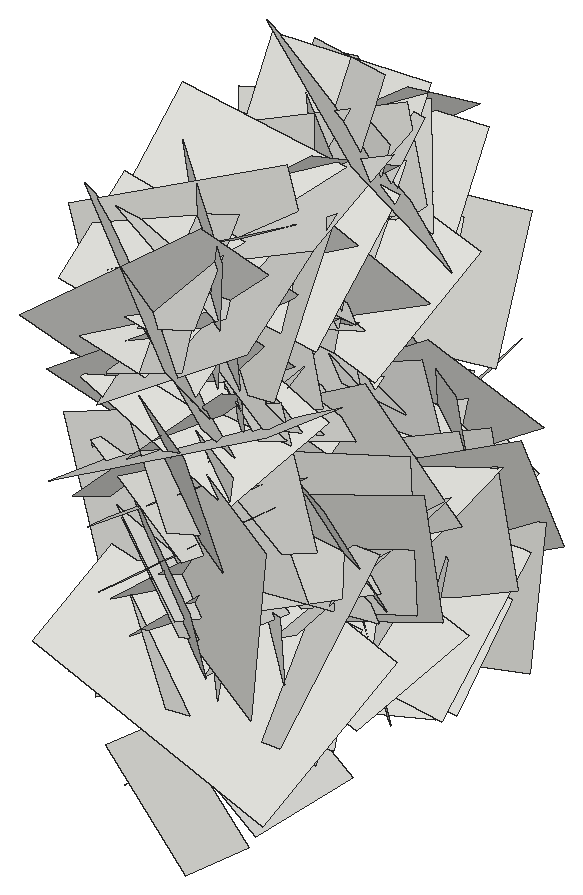
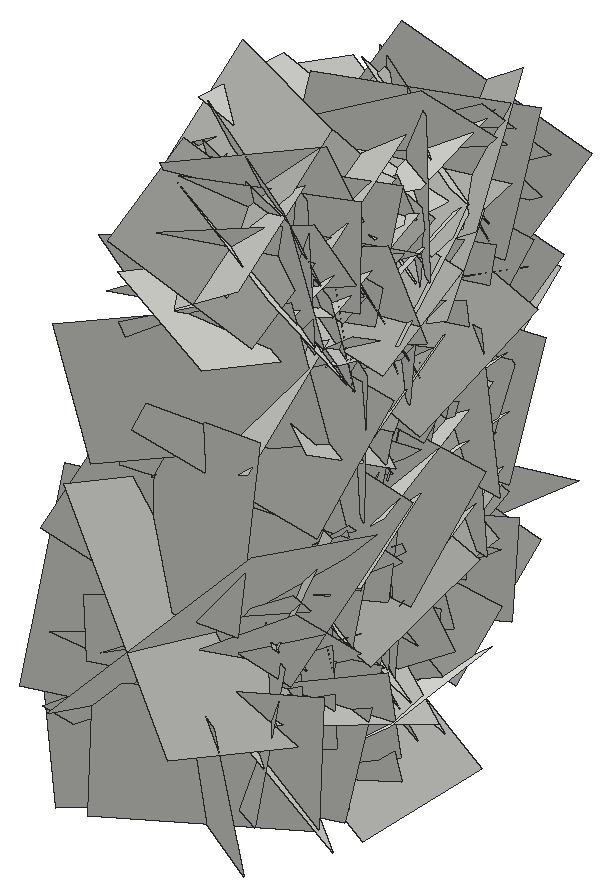
# SketchUp Ruby script. Lengths in inches.
U = 1.inch
M = Sketchup.active_model
def pt(a) = Geom::Point3d.new(a.map { |v| v * U })
def face(e, loops, mat)
  f = e.add_face(loops[0].map { |a| pt(a) })
  loops[1..].each { |l| e.add_face(l.map { |a| pt(a) }).erase! }
  f.material = f.back_material = mat if mat
  f
end
# faces: each face lists its corners as indices into pts; further lists are holes
def faces(e, pts, list, mat = nil) = list.each { |f| face(e, (f[0].is_a?(Array) ? f : [f]).map { |l| l.map { |i| pts[i] } }, mat) }
# xy, xz, yz: faces in a plane at the given z, y or x. An outline is a flat list of corners, or four numbers for a rectangle; further outlines are holes
def ring(l) = l.size == 4 ? [[l[0], l[1]], [l[2], l[1]], [l[2], l[3]], [l[0], l[3]]] : l.each_slice(2).to_a
def flat(e, list, mat, &to3) = list.each { |f| face(e, (f[0].is_a?(Array) ? f : [f]).map { |l| ring(l).map { |u, v| to3.(u, v) } }, mat) }
def xy(e, z, list, mat = nil) = flat(e, list, mat) { |x, y| [x, y, z] }
def xz(e, y, list, mat = nil) = flat(e, list, mat) { |x, z| [x, y, z] }
def yz(e, x, list, mat = nil) = flat(e, list, mat) { |y, z| [x, y, z] }
def lines(e, pts, list) = list.each { |a, b| e.add_line(pt(pts[a]), pt(pts[b])) }
# prism: a flat outline (further loops are holes) pulled along v
def prism(e, loops, v, mat = nil)
  f = face(e, loops, mat); d = Geom::Vector3d.new(v.map { |x| x * U })
  f.pushpull(f.normal.samedirection?(d) ? d.length : -d.length)
end
def box(e, o, s, mat = nil) = prism(e, [[o, [o[0] + s[0], o[1], o[2]], [o[0] + s[0], o[1] + s[1], o[2]], [o[0], o[1] + s[1], o[2]]]], [0, 0, s[2]], mat)
def at(x, y, z, deg = 0) = Geom::Transformation.translation(pt([x, y, z])) * Geom::Transformation.rotation(ORIGIN, Z_AXIS, deg.degrees)
def axes(o, x, y, z) = Geom::Transformation.new([*x, 0, *y, 0, *z, 0, *pt(o).to_a, 1])
def part(name) = M.definitions.add(name)
# library, detail: a bought-in or finely detailed component or shape, given as its bounding box
def library(name, o, s) = part(name).tap { |d| box(d.entities, o, s) }
def detail(e, o, s) = box(e.add_group.entities, o, s)
def put(e, d, t, mat = nil) = e.add_instance(d, t).tap { |i| i.material = mat if mat }
def group(e, t, mat = nil) = e.add_group.tap { |g| g.transformation = t; g.material = mat if mat }.entities
root = M.entities
c1 = part("Component\#6")
p = [[0.01,0,0],[0,3.24,4.54],[4.32,3.24,4.54],[4.33,0,0]]
faces(c1.entities,p,[[0,1,2,3]])
put(root,c1,axes([34.14,198.68,37.125],[0.06347,0.58127,-0.24952],[-0.07215,-0.24326,-0.58302],[0.66662,-0.08167,-0.03935]))
put(root,c1,axes([34.14,193.25,29.42],[-0.0602,0.67546,-0.3863],[-0.10598,-0.39045,-0.66802],[0.81797,-0.00088,-0.11498]))
put(root,c1,axes([34.14,194.71,36.49],[-0.01491,0.71707,-0.22931],[-0.11795,-0.22881,-0.70868],[0.78925,-0.02064,-0.11024]))
put(root,c1,axes([38.11,198.67,35.61],[0.10111,0.59855,0.78971],[-0.15679,0.79307,-0.58323],[-1.03859,-0.06146,0.16492]))
put(root,c1,axes([38.11,206.72,25.52],[0.07134,-1.27871,-0.42932],[0.37284,-0.39835,1.24159],[-1.38032,-0.17369,0.31318]))
put(root,c1,axes([38.11,196.41,37.05],[-0.02372,0.78814,-0.36288],[-0.15491,-0.36124,-0.77556],[-0.90659,0.0411,0.14202]))
put(root,c1,axes([38.11,200.08,36.17],[-0.04967,-0.3024,-0.77978],[-0.15753,-0.76557,0.30582],[-0.87244,0.15545,-0.01082]))
put(root,c1,axes([34.14,194.0625,27.88],[-0.03826,-0.32146,0.75655],[-0.14724,0.74878,0.31153],[0.85881,0.11405,0.08712]))
put(root,c1,axes([34.14,192.62,23.41],[-0.0945,0.05137,0.75973],[0.00531,0.76494,-0.05113],[0.80713,0.00098,0.08928]))
put(root,c1,axes([34.14,194.1,30.97],[-0.07757,0.18705,0.69229],[0.05179,0.69557,-0.18277],[0.75837,-0.02837,0.08329]))
put(root,c1,axes([38.11,192.76,27.5],[0.21382,-0.08753,1.03604],[-0.20559,1.03367,0.1251],[-1.08277,-0.21355,0.18084]))
put(root,c1,axes([34.14,197.11,20.7],[-0.0234,0.20043,0.60552],[0.11848,0.59772,-0.19378],[0.66563,-0.09934,0.05578]))
put(root,c1,axes([38.11,194.12,36.42],[0.16155,0.92195,-0.51802],[-0.06641,-0.51458,-0.93426],[-1.119,0.16364,-0.01934]))
put(root,c1,axes([34.14,192.68,25.51],[0.10584,0.56729,0.32604],[-0.07365,0.33715,-0.56532],[0.68964,-0.05105,-0.11041]))
put(root,c1,axes([38.11,198.72,19.65],[0.06387,-1.04135,0.05905],[0.06023,0.06234,1.04135],[-1.10396,-0.05685,0.06023]))
put(root,c1,axes([38.11,194.92,22.54],[-0.07164,-0.895,0.57486],[0.24411,0.55005,0.88344],[-1.1008,0.18023,0.15849]))
put(root,c1,axes([38.11,200.17,25.9],[-0.12286,-0.34825,-0.84521],[0.12526,-0.85054,0.33424],[-0.96086,-0.06635,0.15165]))
put(root,c1,axes([34.14,196.5,26.6],[-0.00001,0.64808,0.59207],[-0.20568,0.57742,-0.63205],[0.90746,0.13088,-0.14325]))
put(root,c1,axes([38.11,195.45,23.05],[-0.08121,0.42866,0.62692],[-0.16296,0.6083,-0.43472],[-0.78836,-0.1699,0.02528]))
put(root,c1,axes([34.14,201.07,39.9375],[-0.03161,0.68058,-0.41337],[-0.06223,-0.41441,-0.67806],[0.84176,-0.00508,-0.06565]))
put(root,c1,axes([34.14,199.74,34.07],[0.11183,-0.60219,-0.2199],[-0.02555,-0.22643,0.6085],[0.67907,0.09065,0.0591]))
put(root,c1,axes([38.11,195.7,29.31],[0.12944,0.87645,-0.3909],[-0.13192,-0.37627,-0.88251],[-1.00866,0.16168,0.06525]))
put(root,c1,axes([38.11,195.4,26.27],[-0.15303,-0.80886,0.21466],[0.08059,0.20425,0.82078],[-0.8834,0.15875,0.0377]))
put(root,c1,axes([34.14,197.17,21.41],[-0.31691,0.51794,0.91951],[-0.05422,0.94746,-0.55031],[1.11735,0.19287,0.23409]))
put(root,c1,axes([38.11,204.82,25.65],[0.12938,-0.11687,-1.00907],[-0.02351,-1.01639,0.11504],[-1.07651,0.00815,-0.12379]))
put(root,c1,axes([34.14,192.15,39.48],[-0.21361,0.71392,-0.72381],[-0.12034,-0.74908,-0.70723],[1.07091,0.05823,-0.22384]))
put(root,c1,axes([38.11,200.1,34.99],[-0.01875,0.74709,-0.59948],[0.09315,-0.59579,-0.74508],[-1.01106,-0.06874,-0.05753]))
put(root,c1,axes([34.14,198.57,33.25],[-0.09717,0.14422,-0.89801],[-0.11089,-0.89824,-0.13357],[0.95769,-0.08937,-0.10658]))
put(root,c1,axes([38.11,201.91,26.14],[0.02369,0.31708,-0.9382],[0.09459,-0.93526,-0.31396],[-1.04548,-0.07743,-0.04967]))
put(root,c1,axes([38.11,195.16,37.28],[-0.08536,-0.54597,-0.55526],[-0.06407,-0.55215,0.55168],[-0.82294,0.09962,0.01464]))
put(root,c1,axes([34.14,196.95,39.61],[-0.06663,0.78722,-0.39485],[-0.0883,-0.3994,-0.78302],[0.92935,0.01849,-0.10271]))
put(root,c1,axes([34.14,194.17,31.15],[-0.1572,-0.65225,0.62778],[-0.00257,0.63643,0.66066],[0.9596,-0.10514,0.10461]))
put(root,c1,axes([38.11,197.53,26.62],[-0.11622,-0.11144,-0.6986],[-0.08861,-0.69994,0.12478],[-0.74462,0.10068,0.09418]))
put(root,c1,axes([38.11,195.33,34.42],[-0.12228,0.30682,0.85432],[0.19875,0.85067,-0.2802],[-0.94146,0.13973,-0.17012]))
put(root,c1,axes([34.14,195.89,35.57],[-0.03273,-0.74668,0.19464],[0.06894,0.19158,0.74527],[0.81502,-0.04619,-0.05522]))
put(root,c1,axes([34.14,192.38,31.46],[0.05244,0.73173,-0.11131],[0.01157,-0.11227,-0.73318],[0.78447,-0.04726,0.01825]))
put(root,c1,axes([38.11,198.41,25.5],[0.14641,-1.02966,0.26735],[0.10928,0.28128,1.03005],[-1.12233,-0.10694,0.13517]))
put(root,c1,axes([38.11,198.86,35.2],[0.14047,0.16017,0.87964],[-0.13868,0.88315,-0.1411],[-0.93754,-0.10664,0.15267]))
put(root,c1,axes([34.14,193.07,33.95],[0.05953,0.85388,-0.40475],[-0.24794,-0.38029,-0.83472],[0.97048,-0.14953,-0.18843]))
put(root,c1,axes([34.14,201.02,39.48],[-0.13577,0.09163,-0.9618],[-0.05798,-0.96935,-0.08506],[1.02248,-0.0428,-0.13253]))
put(root,c1,axes([34.14,192.92,34.17],[-0.15147,-0.1521,1.01718],[-0.1212,1.02293,0.1369],[1.08344,0.09316,0.15752]))
put(root,c1,axes([38.11,191.375,35.34],[-0.1473,0.40574,0.51918],[-0.07991,0.51733,-0.42447],[-0.69387,-0.14571,-0.06134]))
put(root,c1,axes([38.11,194.18,31.13],[0.04063,-0.16003,0.87853],[0.02386,0.87924,0.15917],[-0.94627,0.0153,0.04174]))
put(root,c1,axes([34.14,202.06,39.63],[-0.00244,-0.36914,-0.6705],[0.07457,-0.66776,0.36739],[0.80789,0.06052,-0.03594]))
put(root,c1,axes([38.11,201.02,32],[0.03236,-0.79816,-0.43551],[0.07074,-0.43262,0.79753],[-0.9612,-0.0587,0.04403]))
put(root,c1,axes([38.11,199.18,25.47],[-0.11604,-0.3767,0.6399],[0.02749,0.64448,0.38383],[-0.78661,0.07809,-0.08099]))
put(root,c1,axes([34.14,199.18,25.47],[0.11604,-0.3767,0.6399],[-0.02749,0.64448,0.38383],[0.78661,0.07809,-0.08099]))
put(root,c1,axes([34.14,201.02,32],[-0.03236,-0.79816,-0.43551],[-0.07074,-0.43262,0.79753],[0.9612,-0.0587,0.04403]))
put(root,c1,axes([38.11,202.06,39.63],[0.00244,-0.36914,-0.6705],[-0.07457,-0.66776,0.36739],[-0.80789,0.06052,-0.03594]))
put(root,c1,axes([34.14,194.18,31.13],[-0.04063,-0.16003,0.87853],[-0.02386,0.87924,0.15917],[0.94627,0.0153,0.04174]))
put(root,c1,axes([34.14,191.375,35.34],[0.1473,0.40574,0.51918],[0.07991,0.51733,-0.42447],[0.69387,-0.14571,-0.06134]))
put(root,c1,axes([38.11,192.92,34.17],[0.15147,-0.1521,1.01718],[0.1212,1.02293,0.1369],[-1.08344,0.09316,0.15752]))
put(root,c1,axes([38.11,201.02,39.48],[0.13577,0.09163,-0.9618],[0.05798,-0.96935,-0.08506],[-1.02248,-0.0428,-0.13253]))
put(root,c1,axes([38.11,193.07,33.95],[-0.05953,0.85388,-0.40475],[0.24794,-0.38029,-0.83472],[-0.97048,-0.14953,-0.18843]))
put(root,c1,axes([34.14,198.86,35.2],[-0.14047,0.16017,0.87964],[0.13868,0.88315,-0.1411],[0.93754,-0.10664,0.15267]))
put(root,c1,axes([34.14,198.41,25.5],[-0.14641,-1.02966,0.26735],[-0.10928,0.28128,1.03005],[1.12233,-0.10694,0.13517]))
put(root,c1,axes([38.11,192.38,31.46],[-0.05244,0.73173,-0.11131],[-0.01157,-0.11227,-0.73318],[-0.78447,-0.04726,0.01825]))
put(root,c1,axes([38.11,195.89,35.57],[0.03273,-0.74668,0.19464],[-0.06894,0.19158,0.74527],[-0.81502,-0.04619,-0.05522]))
put(root,c1,axes([34.14,195.33,34.42],[0.12228,0.30682,0.85432],[-0.19875,0.85067,-0.2802],[0.94146,0.13973,-0.17012]))
put(root,c1,axes([34.14,197.53,26.62],[0.11622,-0.11144,-0.6986],[0.08861,-0.69994,0.12478],[0.74462,0.10068,0.09418]))
put(root,c1,axes([38.11,194.17,31.15],[0.1572,-0.65225,0.62778],[0.00257,0.63643,0.66066],[-0.9596,-0.10514,0.10461]))
put(root,c1,axes([38.11,196.95,39.61],[0.06663,0.78722,-0.39485],[0.0883,-0.3994,-0.78302],[-0.92935,0.01849,-0.10271]))
put(root,c1,axes([34.14,195.16,37.28],[0.08536,-0.54597,-0.55526],[0.06407,-0.55215,0.55168],[0.82294,0.09962,0.01464]))
put(root,c1,axes([34.14,201.91,26.14],[-0.02369,0.31708,-0.9382],[-0.09459,-0.93526,-0.31396],[1.04548,-0.07743,-0.04967]))
put(root,c1,axes([38.11,198.57,33.25],[0.09717,0.14422,-0.89801],[0.11089,-0.89824,-0.13357],[-0.95769,-0.08937,-0.10658]))
put(root,c1,axes([34.14,200.1,34.99],[0.01875,0.74709,-0.59948],[-0.09315,-0.59579,-0.74508],[1.01106,-0.06874,-0.05753]))
put(root,c1,axes([38.11,192.15,39.48],[0.21361,0.71392,-0.72381],[0.12034,-0.74908,-0.70723],[-1.07091,0.05823,-0.22384]))
put(root,c1,axes([34.14,204.82,25.65],[-0.12938,-0.11687,-1.00907],[0.02351,-1.01639,0.11504],[1.07651,0.00815,-0.12379]))
put(root,c1,axes([38.11,197.17,21.41],[0.31691,0.51794,0.91951],[0.05422,0.94746,-0.55031],[-1.11735,0.19287,0.23409]))
put(root,c1,axes([34.14,195.4,26.27],[0.15303,-0.80886,0.21466],[-0.08059,0.20425,0.82078],[0.8834,0.15875,0.0377]))
put(root,c1,axes([34.14,195.7,29.31],[-0.12944,0.87645,-0.3909],[0.13192,-0.37627,-0.88251],[1.00866,0.16168,0.06525]))
put(root,c1,axes([38.11,199.74,34.07],[-0.11183,-0.60219,-0.2199],[0.02555,-0.22643,0.6085],[-0.67907,0.09065,0.0591]))
put(root,c1,axes([38.11,201.07,39.9375],[0.03161,0.68058,-0.41337],[0.06223,-0.41441,-0.67806],[-0.84176,-0.00508,-0.06565]))
put(root,c1,axes([34.14,195.45,23.05],[0.08121,0.42866,0.62692],[0.16296,0.6083,-0.43472],[0.78836,-0.1699,0.02528]))
put(root,c1,axes([38.11,196.5,26.6],[0.00001,0.64808,0.59207],[0.20568,0.57742,-0.63205],[-0.90746,0.13088,-0.14325]))
put(root,c1,axes([34.14,200.17,25.9],[0.12286,-0.34825,-0.84521],[-0.12526,-0.85054,0.33424],[0.96086,-0.06635,0.15165]))
put(root,c1,axes([34.14,194.92,22.54],[0.07164,-0.895,0.57486],[-0.24411,0.55005,0.88344],[1.1008,0.18023,0.15849]))
put(root,c1,axes([34.14,198.72,19.65],[-0.06387,-1.04135,0.05905],[-0.06023,0.06234,1.04135],[1.10396,-0.05685,0.06023]))
put(root,c1,axes([38.11,192.68,25.51],[-0.10584,0.56729,0.32604],[0.07365,0.33715,-0.56532],[-0.68964,-0.05105,-0.11041]))
put(root,c1,axes([34.14,194.12,36.42],[-0.16155,0.92195,-0.51802],[0.06641,-0.51458,-0.93426],[1.119,0.16364,-0.01934]))
put(root,c1,axes([38.11,197.11,20.7],[0.0234,0.20043,0.60552],[-0.11848,0.59772,-0.19378],[-0.66563,-0.09934,0.05578]))
put(root,c1,axes([34.14,192.76,27.5],[-0.21382,-0.08753,1.03604],[0.20559,1.03367,0.1251],[1.08277,-0.21355,0.18084]))
put(root,c1,axes([38.11,194.1,30.97],[0.07757,0.18705,0.69229],[-0.05179,0.69557,-0.18277],[-0.75837,-0.02837,0.08329]))
put(root,c1,axes([38.11,192.62,23.41],[0.0945,0.05137,0.75973],[-0.00531,0.76494,-0.05113],[-0.80713,0.00098,0.08928]))
put(root,c1,axes([38.11,194.0625,27.88],[0.03826,-0.32146,0.75655],[0.14724,0.74878,0.31153],[-0.85881,0.11405,0.08712]))
put(root,c1,axes([34.14,200.08,36.17],[0.04967,-0.3024,-0.77978],[0.15753,-0.76557,0.30582],[0.87244,0.15545,-0.01082]))
put(root,c1,axes([34.14,196.41,37.05],[0.02372,0.78814,-0.36288],[0.15491,-0.36124,-0.77556],[0.90659,0.0411,0.14202]))
put(root,c1,axes([34.14,206.72,25.52],[-0.07134,-1.27871,-0.42932],[-0.37284,-0.39835,1.24159],[1.38032,-0.17369,0.31318]))
put(root,c1,axes([34.14,198.67,35.61],[-0.10111,0.59855,0.78971],[0.15679,0.79307,-0.58323],[1.03859,-0.06146,0.16492]))
put(root,c1,axes([38.11,194.71,36.49],[0.01491,0.71707,-0.22931],[0.11795,-0.22881,-0.70868],[-0.78925,-0.02064,-0.11024]))
put(root,c1,axes([38.11,193.25,29.42],[0.0602,0.67546,-0.3863],[0.10598,-0.39045,-0.66802],[-0.81797,-0.00088,-0.11498]))
put(root,c1,axes([38.11,198.68,37.125],[-0.06347,0.58127,-0.24952],[0.07215,-0.24326,-0.58302],[-0.66662,-0.08167,-0.03935]))
put(root,c1,axes([34.14,195.125,35.61],[0.03117,0.92717,-0.40656],[-0.02653,-0.40594,-0.92757],[1.07281,-0.03698,-0.01113]))
put(root,c1,axes([38.11,200.57,36.04],[0.10099,0.61602,0.17436],[-0.1325,0.19079,-0.60575],[-0.66557,0.05549,0.14705]))
put(root,c1,axes([34.14,197.34,38.49],[0.22162,0.66132,-0.53694],[-0.02723,-0.54773,-0.68462],[0.90256,-0.17891,0.1112]))
put(root,c1,axes([34.14,198.8,27.02],[-0.0226,-0.2767,0.96977],[0.06915,0.96758,0.27751],[1.06674,-0.06859,0.00256]))
put(root,c1,axes([34.14,193.58,33.2],[0.1306,0.22319,-0.86205],[0.05382,-0.87061,-0.21815],[0.94237,0.01879,0.13193]))
put(root,c1,axes([34.14,197.85,24.73],[-0.35143,-0.52734,1.13432],[0.18025,1.14359,0.58135],[1.31365,-0.29799,0.22369]))
put(root,c1,axes([38.11,196.3,29.33],[0.09147,0.43894,-0.4809],[-0.05464,-0.47898,-0.44644],[-0.688,0.09639,-0.02848]))
put(root,c1,axes([38.11,192.39,25.48],[0.15082,-0.34829,0.66058],[0.01541,0.67363,0.35204],[-0.79143,-0.05326,0.13274]))
put(root,c1,axes([34.14,199.8,22.82],[-0.00598,0.07204,1.08492],[-0.02761,1.08461,-0.07215],[1.15221,0.02636,0.0039]))
put(root,c1,axes([38.11,194.26,19.42],[0.05867,-0.70774,0.13488],[0.12622,0.14241,0.69835],[-0.75321,-0.03127,0.12754]))
put(root,c1,axes([34.14,196.22,30.25],[-0.08073,-0.93811,0.99109],[-0.27356,0.98462,0.91216],[1.42044,0.13631,0.232]))
put(root,c1,axes([34.14,191.97,33.56],[0.08688,0.89449,0.25558],[0.12211,0.24484,-0.89383],[0.97851,-0.10998,0.08885]))
put(root,c1,axes([34.14,197.83,24.35],[-0.09568,0.96283,0.81475],[-0.1112,0.80827,-0.9668],[1.33234,0.1366,-0.02218]))
put(root,c1,axes([34.14,199.05,27.98],[0.08019,0.19915,0.92966],[0.13728,0.92174,-0.20799],[0.9984,-0.14274,-0.04607]))
put(root,c1,axes([34.14,202.95,33.21],[-0.17447,0.42234,-1.07867],[0.17991,-1.06896,-0.44444],[1.21466,0.21899,-0.08911]))
put(root,c1,axes([34.14,201.66,25.46],[-0.21728,-0.88431,0.94199],[0.03627,0.94972,0.89901],[1.36907,-0.16551,0.12568]))
put(root,c1,axes([34.14,195.04,27.27],[0.2131,0.57774,0.71728],[0.02179,0.73117,-0.59469],[0.97604,-0.14247,-0.14333]))
put(root,c1,axes([34.14,197.22,25.56],[0.17769,-0.12121,-0.94504],[0.07151,-0.95564,0.13453],[1.00742,0.08922,0.15714]))
put(root,c1,axes([34.14,192.77,37.47],[-0.01566,0.85002,0.74451],[0.07038,0.74394,-0.84805],[1.19569,-0.03266,0.05967]))
put(root,c1,axes([38.11,203.75,35.72],[0.12855,-0.35471,-0.52952],[0.05195,-0.53223,0.36775],[-0.67359,-0.10874,-0.07269]))
put(root,c1,axes([34.14,202.23,24.6],[-0.19755,-1.2824,-0.48224],[-0.04087,-0.48158,1.29554],[1.4517,-0.18807,-0.02915]))
put(root,c1,axes([34.14,200.11,31.93],[0.08158,0.26048,1.04137],[0.05734,1.04178,-0.26458],[1.13642,-0.07126,-0.06141]))
put(root,c1,axes([34.14,198.78,35.93],[0.06513,-0.64723,-0.92238],[0.00055,-0.92374,0.64822],[1.19442,0.03572,0.05]))
put(root,c1,axes([34.14,196.35,35.86],[0.06555,0.97369,0.5362],[0.0688,0.53295,-0.97527],[1.17625,-0.08544,0.02716]))
put(root,c1,axes([34.14,195.34,33.06],[0.01901,1.14103,-0.72029],[-0.19621,-0.71146,-1.13165],[1.41679,-0.11384,-0.14706]))
put(root,c1,axes([34.14,197.73,24.08],[0.06299,0.80841,0.87356],[-0.01823,0.87514,-0.8087],[1.26151,-0.02772,-0.0553]))
put(root,c1,axes([34.14,194.3,32.47],[-0.23408,0.14056,-1.33491],[0.22407,-1.33233,-0.17526],[1.40507,0.23589,-0.19445]))
put(root,c1,axes([34.14,196.04,25.17],[0.02819,1.07686,0.22249],[0.25409,0.21152,-1.05244],[1.13755,-0.07393,0.22957]))
put(root,c1,axes([34.14,193.85,32.27],[0.12737,1.17977,-0.33684],[-0.1012,-0.32843,-1.18439],[1.29659,-0.14153,-0.05935]))
put(root,c1,axes([34.14,198.24,37.08],[0.15669,-0.99926,-0.19378],[0.22295,-0.1616,0.99377],[1.05566,0.18244,-0.18112]))
put(root,c1,axes([34.14,197.21,31.46],[0.04455,0.58157,-0.95839],[0.2239,-0.94599,-0.56478],[1.16701,0.1593,0.14494]))
put(root,c1,axes([34.14,200.75,21.625],[0.14431,-0.01788,1.13958],[0.06693,1.14604,0.01044],[1.20625,-0.06145,-0.13692]))
put(root,c1,axes([34.14,198.29,23.22],[0.04433,-0.32511,1.32538],[-0.126,1.3201,0.32757],[1.44106,0.12543,-0.01213]))
put(root,c1,axes([34.14,196.35,30.1],[0.25467,1.00338,0.64071],[-0.12934,0.67094,-1.00496],[1.25528,-0.13443,-0.23354]))
put(root,c1,axes([34.14,199.72,26.12],[-0.08735,-0.8928,-1.02237],[0.07635,-1.02569,0.88989],[1.43674,0.00023,-0.10945]))
put(root,c1,axes([34.14,196.54,35.06],[0.17609,-1.11494,-0.45613],[-0.00034,-0.46049,1.12547],[1.27691,0.15363,0.0632]))
put(root,c1,axes([34.14,189.88,26.35],[0.12674,1.17916,0.69894],[-0.07675,0.70605,-1.17877],[1.45096,-0.06565,-0.1234]))
put(root,c1,axes([34.14,194.52,25.48],[0.11423,-0.20624,1.26777],[0.06819,1.2715,0.20138],[1.3598,-0.04643,-0.1166]))
put(root,c1,axes([34.14,193.84,30.46],[0.25587,-1.06575,0.3461],[0.15582,0.3811,1.07099],[1.17751,0.18115,-0.21693]))
put(root,c1,axes([34.14,199.97,41.09],[0.2759,0.65189,-0.94787],[0.07756,-0.97924,-0.65337],[1.21695,-0.08538,0.25653]))
put(root,c1,axes([34.14,200.57,23.13],[0.2198,-0.69796,1.13548],[-0.0671,1.14269,0.71395],[1.41122,0.16304,-0.1429]))
put(root,c1,axes([34.14,195.625,24.52],[0.22176,-0.47224,1.18941],[0.10161,1.2076,0.46259],[1.3527,-0.0133,-0.22974]))
